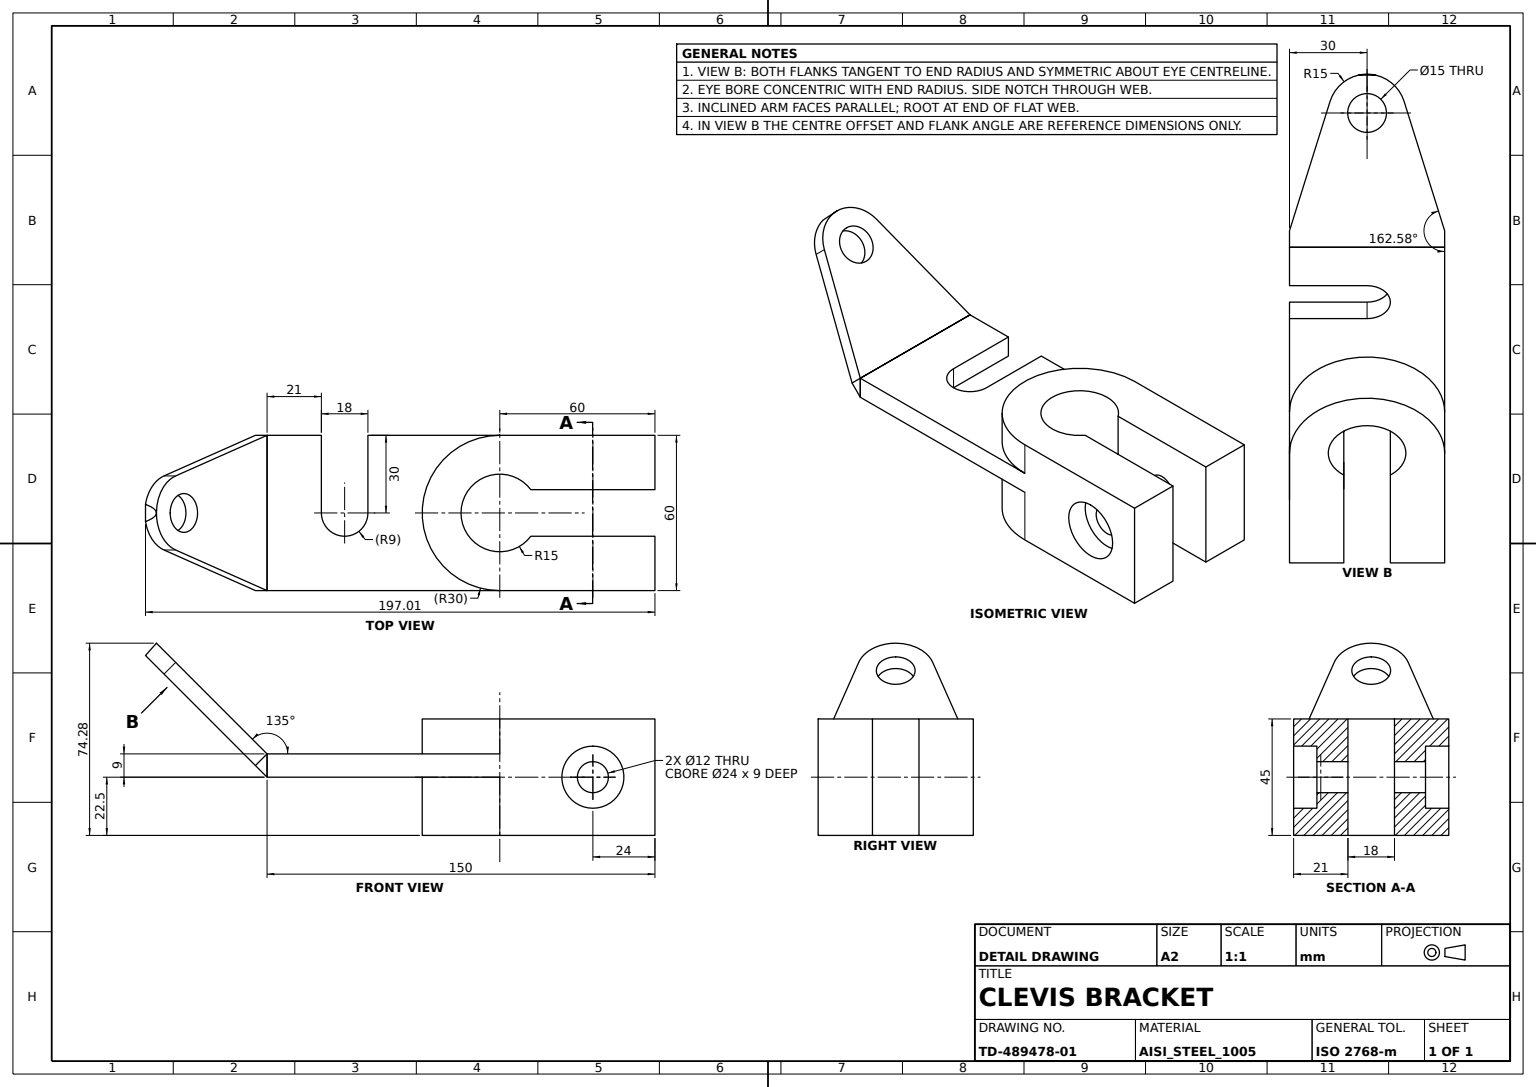
ISO-10303-21;
HEADER;
FILE_DESCRIPTION((''),'2;1');
FILE_NAME('','',(''),(''),'','','');
FILE_SCHEMA(('AUTOMOTIVE_DESIGN'));
ENDSEC;
DATA;
#1=APPLICATION_CONTEXT('');
#2=PRODUCT_CONTEXT('',#1,'mechanical');
#3=PRODUCT('','','',(#2));
#4=PRODUCT_DEFINITION_FORMATION('','',#3);
#5=PRODUCT_DEFINITION_CONTEXT('',#1,'design');
#6=PRODUCT_DEFINITION('','',#4,#5);
#7=PRODUCT_DEFINITION_SHAPE('','',#6);
#8=(LENGTH_UNIT()NAMED_UNIT(*)SI_UNIT(.MILLI.,.METRE.));
#9=(NAMED_UNIT(*)PLANE_ANGLE_UNIT()SI_UNIT($,.RADIAN.));
#10=(NAMED_UNIT(*)SI_UNIT($,.STERADIAN.)SOLID_ANGLE_UNIT());
#11=UNCERTAINTY_MEASURE_WITH_UNIT(LENGTH_MEASURE(0.005),#8,'distance_accuracy_value','');
#12=(GEOMETRIC_REPRESENTATION_CONTEXT(3)GLOBAL_UNCERTAINTY_ASSIGNED_CONTEXT((#11))GLOBAL_UNIT_ASSIGNED_CONTEXT((#8,#9,#10))REPRESENTATION_CONTEXT('',''));
#13=CARTESIAN_POINT('',(-90.,-30.,9.));
#14=VERTEX_POINT('',#13);
#15=CARTESIAN_POINT('',(-90.,30.,9.));
#16=VERTEX_POINT('',#15);
#17=DIRECTION('',(0.,1.,0.));
#18=VECTOR('',#17,1000.);
#19=LINE('',#13,#18);
#20=EDGE_CURVE('',#14,#16,#19,.T.);
#21=ORIENTED_EDGE('',*,*,#20,.F.);
#22=CARTESIAN_POINT('',(0.,-30.,9.));
#23=VERTEX_POINT('',#22);
#24=DIRECTION('',(-1.,0.,0.));
#25=VECTOR('',#24,1000.);
#26=LINE('',#22,#25);
#27=EDGE_CURVE('',#23,#14,#26,.T.);
#28=ORIENTED_EDGE('',*,*,#27,.F.);
#29=CARTESIAN_POINT('',(0.,30.,9.));
#30=VERTEX_POINT('',#29);
#31=CARTESIAN_POINT('',(0.,0.,9.));
#32=DIRECTION('',(0.,0.,1.));
#33=DIRECTION('',(1.,0.,0.));
#34=AXIS2_PLACEMENT_3D('',#31,#32,#33);
#35=CIRCLE('',#34,30.);
#36=EDGE_CURVE('',#30,#23,#35,.T.);
#37=ORIENTED_EDGE('',*,*,#36,.F.);
#38=CARTESIAN_POINT('',(-51.,30.,9.));
#39=VERTEX_POINT('',#38);
#40=VECTOR('',#33,1000.);
#41=LINE('',#38,#40);
#42=EDGE_CURVE('',#39,#30,#41,.T.);
#43=ORIENTED_EDGE('',*,*,#42,.F.);
#44=CARTESIAN_POINT('',(-51.,0.,9.));
#45=VERTEX_POINT('',#44);
#46=LINE('',#44,#18);
#47=EDGE_CURVE('',#45,#39,#46,.T.);
#48=ORIENTED_EDGE('',*,*,#47,.F.);
#49=CARTESIAN_POINT('',(-69.,0.,9.));
#50=VERTEX_POINT('',#49);
#51=CARTESIAN_POINT('',(-60.,0.,9.));
#52=AXIS2_PLACEMENT_3D('',#51,#32,#33);
#53=CIRCLE('',#52,9.);
#54=EDGE_CURVE('',#50,#45,#53,.T.);
#55=ORIENTED_EDGE('',*,*,#54,.F.);
#56=CARTESIAN_POINT('',(-69.,30.,9.));
#57=VERTEX_POINT('',#56);
#58=DIRECTION('',(0.,-1.,0.));
#59=VECTOR('',#58,1000.);
#60=LINE('',#56,#59);
#61=EDGE_CURVE('',#57,#50,#60,.T.);
#62=ORIENTED_EDGE('',*,*,#61,.F.);
#63=LINE('',#15,#40);
#64=EDGE_CURVE('',#16,#57,#63,.T.);
#65=ORIENTED_EDGE('',*,*,#64,.F.);
#66=EDGE_LOOP('',(#21,#28,#37,#43,#48,#55,#62,#65));
#67=FACE_BOUND('',#66,.T.);
#68=PLANE('',#52);
#69=ADVANCED_FACE('',(#67),#68,.T.);
#70=CARTESIAN_POINT('',(60.,-30.,22.5));
#71=VERTEX_POINT('',#70);
#72=CARTESIAN_POINT('',(60.,-30.,-22.5));
#73=VERTEX_POINT('',#72);
#74=DIRECTION('',(0.,0.,-1.));
#75=VECTOR('',#74,1000.);
#76=LINE('',#70,#75);
#77=EDGE_CURVE('',#71,#73,#76,.T.);
#78=ORIENTED_EDGE('',*,*,#77,.T.);
#79=CARTESIAN_POINT('',(60.,-9.,-22.5));
#80=VERTEX_POINT('',#79);
#81=LINE('',#72,#18);
#82=EDGE_CURVE('',#73,#80,#81,.T.);
#83=ORIENTED_EDGE('',*,*,#82,.T.);
#84=CARTESIAN_POINT('',(60.,-9.,22.5));
#85=VERTEX_POINT('',#84);
#86=LINE('',#84,#75);
#87=EDGE_CURVE('',#85,#80,#86,.T.);
#88=ORIENTED_EDGE('',*,*,#87,.F.);
#89=LINE('',#70,#18);
#90=EDGE_CURVE('',#71,#85,#89,.T.);
#91=ORIENTED_EDGE('',*,*,#90,.F.);
#92=EDGE_LOOP('',(#78,#83,#88,#91));
#93=FACE_BOUND('',#92,.T.);
#94=AXIS2_PLACEMENT_3D('',#70,#24,#58);
#95=PLANE('',#94);
#96=ADVANCED_FACE('',(#93),#95,.F.);
#97=CARTESIAN_POINT('',(36.,21.,-12.));
#98=VERTEX_POINT('',#97);
#99=CARTESIAN_POINT('',(36.,21.,0.));
#100=AXIS2_PLACEMENT_3D('',#99,#58,#74);
#101=CIRCLE('',#100,12.);
#102=EDGE_CURVE('',#98,#98,#101,.T.);
#103=ORIENTED_EDGE('',*,*,#102,.T.);
#104=EDGE_LOOP('',(#103));
#105=FACE_BOUND('',#104,.T.);
#106=CARTESIAN_POINT('',(36.,30.,-12.));
#107=VERTEX_POINT('',#106);
#108=CARTESIAN_POINT('',(36.,30.,0.));
#109=AXIS2_PLACEMENT_3D('',#108,#58,#74);
#110=CIRCLE('',#109,12.);
#111=EDGE_CURVE('',#107,#107,#110,.T.);
#112=ORIENTED_EDGE('',*,*,#111,.F.);
#113=EDGE_LOOP('',(#112));
#114=FACE_BOUND('',#113,.T.);
#115=CYLINDRICAL_SURFACE('',#109,12.);
#116=ADVANCED_FACE('',(#105,#114),#115,.F.);
#117=ORIENTED_EDGE('',*,*,#64,.T.);
#118=CARTESIAN_POINT('',(-69.,30.,0.));
#119=VERTEX_POINT('',#118);
#120=LINE('',#56,#75);
#121=EDGE_CURVE('',#57,#119,#120,.T.);
#122=ORIENTED_EDGE('',*,*,#121,.T.);
#123=CARTESIAN_POINT('',(-90.,30.,0.));
#124=VERTEX_POINT('',#123);
#125=LINE('',#123,#40);
#126=EDGE_CURVE('',#124,#119,#125,.T.);
#127=ORIENTED_EDGE('',*,*,#126,.F.);
#128=LINE('',#15,#75);
#129=EDGE_CURVE('',#16,#124,#128,.T.);
#130=ORIENTED_EDGE('',*,*,#129,.F.);
#131=EDGE_LOOP('',(#117,#122,#127,#130));
#132=FACE_BOUND('',#131,.T.);
#133=AXIS2_PLACEMENT_3D('',#15,#17,#24);
#134=PLANE('',#133);
#135=ADVANCED_FACE('',(#132),#134,.T.);
#136=CARTESIAN_POINT('',(36.,9.,6.));
#137=VERTEX_POINT('',#136);
#138=CARTESIAN_POINT('',(36.,9.,0.));
#139=AXIS2_PLACEMENT_3D('',#138,#17,#32);
#140=CIRCLE('',#139,6.);
#141=EDGE_CURVE('',#137,#137,#140,.T.);
#142=ORIENTED_EDGE('',*,*,#141,.F.);
#143=EDGE_LOOP('',(#142));
#144=FACE_BOUND('',#143,.T.);
#145=CARTESIAN_POINT('',(36.,21.,-6.));
#146=VERTEX_POINT('',#145);
#147=CIRCLE('',#100,6.);
#148=EDGE_CURVE('',#146,#146,#147,.T.);
#149=ORIENTED_EDGE('',*,*,#148,.F.);
#150=EDGE_LOOP('',(#149));
#151=FACE_BOUND('',#150,.T.);
#152=CARTESIAN_POINT('',(36.,-60.916439,0.));
#153=AXIS2_PLACEMENT_3D('',#152,#58,#74);
#154=CYLINDRICAL_SURFACE('',#153,6.);
#155=ADVANCED_FACE('',(#144,#151),#154,.F.);
#156=CARTESIAN_POINT('',(36.,-30.,12.));
#157=VERTEX_POINT('',#156);
#158=CARTESIAN_POINT('',(36.,-30.,0.));
#159=AXIS2_PLACEMENT_3D('',#158,#17,#32);
#160=CIRCLE('',#159,12.);
#161=EDGE_CURVE('',#157,#157,#160,.T.);
#162=ORIENTED_EDGE('',*,*,#161,.F.);
#163=EDGE_LOOP('',(#162));
#164=FACE_BOUND('',#163,.T.);
#165=CARTESIAN_POINT('',(36.,-21.,12.));
#166=VERTEX_POINT('',#165);
#167=CARTESIAN_POINT('',(36.,-21.,0.));
#168=AXIS2_PLACEMENT_3D('',#167,#17,#32);
#169=CIRCLE('',#168,12.);
#170=EDGE_CURVE('',#166,#166,#169,.F.);
#171=ORIENTED_EDGE('',*,*,#170,.F.);
#172=EDGE_LOOP('',(#171));
#173=FACE_BOUND('',#172,.T.);
#174=CYLINDRICAL_SURFACE('',#159,12.);
#175=ADVANCED_FACE('',(#164,#173),#174,.F.);
#176=CARTESIAN_POINT('',(0.,30.,-22.5));
#177=VERTEX_POINT('',#176);
#178=CARTESIAN_POINT('',(0.,-30.,-22.5));
#179=VERTEX_POINT('',#178);
#180=CARTESIAN_POINT('',(0.,0.,-22.5));
#181=AXIS2_PLACEMENT_3D('',#180,#32,#33);
#182=CIRCLE('',#181,30.);
#183=EDGE_CURVE('',#177,#179,#182,.T.);
#184=ORIENTED_EDGE('',*,*,#183,.T.);
#185=CARTESIAN_POINT('',(0.,-30.,0.));
#186=VERTEX_POINT('',#185);
#187=CARTESIAN_POINT('',(0.,-30.,22.5));
#188=LINE('',#187,#75);
#189=EDGE_CURVE('',#186,#179,#188,.T.);
#190=ORIENTED_EDGE('',*,*,#189,.F.);
#191=CARTESIAN_POINT('',(0.,30.,0.));
#192=VERTEX_POINT('',#191);
#193=CARTESIAN_POINT('',(0.,0.,0.));
#194=AXIS2_PLACEMENT_3D('',#193,#32,#33);
#195=CIRCLE('',#194,30.);
#196=EDGE_CURVE('',#192,#186,#195,.T.);
#197=ORIENTED_EDGE('',*,*,#196,.F.);
#198=CARTESIAN_POINT('',(0.,30.,22.5));
#199=LINE('',#198,#75);
#200=EDGE_CURVE('',#192,#177,#199,.T.);
#201=ORIENTED_EDGE('',*,*,#200,.T.);
#202=EDGE_LOOP('',(#184,#190,#197,#201));
#203=FACE_BOUND('',#202,.T.);
#204=CARTESIAN_POINT('',(0.,0.,22.5));
#205=AXIS2_PLACEMENT_3D('',#204,#74,#24);
#206=CYLINDRICAL_SURFACE('',#205,30.);
#207=ADVANCED_FACE('',(#203),#206,.T.);
#208=ORIENTED_EDGE('',*,*,#102,.F.);
#209=EDGE_LOOP('',(#208));
#210=FACE_BOUND('',#209,.T.);
#211=ORIENTED_EDGE('',*,*,#148,.T.);
#212=EDGE_LOOP('',(#211));
#213=FACE_BOUND('',#212,.T.);
#214=PLANE('',#100);
#215=ADVANCED_FACE('',(#210,#213),#214,.F.);
#216=ORIENTED_EDGE('',*,*,#170,.T.);
#217=EDGE_LOOP('',(#216));
#218=FACE_BOUND('',#217,.T.);
#219=CARTESIAN_POINT('',(36.,-21.,6.));
#220=VERTEX_POINT('',#219);
#221=CIRCLE('',#168,6.);
#222=EDGE_CURVE('',#220,#220,#221,.F.);
#223=ORIENTED_EDGE('',*,*,#222,.F.);
#224=EDGE_LOOP('',(#223));
#225=FACE_BOUND('',#224,.T.);
#226=PLANE('',#168);
#227=ADVANCED_FACE('',(#218,#225),#226,.F.);
#228=CARTESIAN_POINT('',(12.,9.,22.5));
#229=VERTEX_POINT('',#228);
#230=CARTESIAN_POINT('',(60.,9.,22.5));
#231=VERTEX_POINT('',#230);
#232=LINE('',#228,#40);
#233=EDGE_CURVE('',#229,#231,#232,.T.);
#234=ORIENTED_EDGE('',*,*,#233,.T.);
#235=CARTESIAN_POINT('',(60.,30.,22.5));
#236=VERTEX_POINT('',#235);
#237=LINE('',#230,#18);
#238=EDGE_CURVE('',#231,#236,#237,.T.);
#239=ORIENTED_EDGE('',*,*,#238,.T.);
#240=VERTEX_POINT('',#198);
#241=LINE('',#235,#25);
#242=EDGE_CURVE('',#236,#240,#241,.T.);
#243=ORIENTED_EDGE('',*,*,#242,.T.);
#244=VERTEX_POINT('',#187);
#245=AXIS2_PLACEMENT_3D('',#204,#32,#33);
#246=CIRCLE('',#245,30.);
#247=EDGE_CURVE('',#240,#244,#246,.T.);
#248=ORIENTED_EDGE('',*,*,#247,.T.);
#249=LINE('',#187,#40);
#250=EDGE_CURVE('',#244,#71,#249,.T.);
#251=ORIENTED_EDGE('',*,*,#250,.T.);
#252=ORIENTED_EDGE('',*,*,#90,.T.);
#253=CARTESIAN_POINT('',(12.,-9.,22.5));
#254=VERTEX_POINT('',#253);
#255=LINE('',#84,#25);
#256=EDGE_CURVE('',#85,#254,#255,.T.);
#257=ORIENTED_EDGE('',*,*,#256,.T.);
#258=AXIS2_PLACEMENT_3D('',#204,#74,#33);
#259=CIRCLE('',#258,15.);
#260=EDGE_CURVE('',#254,#229,#259,.T.);
#261=ORIENTED_EDGE('',*,*,#260,.T.);
#262=EDGE_LOOP('',(#234,#239,#243,#248,#251,#252,#257,#261));
#263=FACE_BOUND('',#262,.T.);
#264=PLANE('',#245);
#265=ADVANCED_FACE('',(#263),#264,.T.);
#266=ORIENTED_EDGE('',*,*,#20,.T.);
#267=ORIENTED_EDGE('',*,*,#129,.T.);
#268=CARTESIAN_POINT('',(-90.,-30.,0.));
#269=VERTEX_POINT('',#268);
#270=LINE('',#268,#18);
#271=EDGE_CURVE('',#269,#124,#270,.T.);
#272=ORIENTED_EDGE('',*,*,#271,.F.);
#273=LINE('',#13,#75);
#274=EDGE_CURVE('',#14,#269,#273,.T.);
#275=ORIENTED_EDGE('',*,*,#274,.F.);
#276=EDGE_LOOP('',(#266,#267,#272,#275));
#277=FACE_BOUND('',#276,.T.);
#278=AXIS2_PLACEMENT_3D('',#13,#24,#32);
#279=PLANE('',#278);
#280=ADVANCED_FACE('',(#277),#279,.T.);
#281=CARTESIAN_POINT('',(12.,9.,-22.5));
#282=VERTEX_POINT('',#281);
#283=LINE('',#228,#75);
#284=EDGE_CURVE('',#229,#282,#283,.T.);
#285=ORIENTED_EDGE('',*,*,#284,.T.);
#286=CARTESIAN_POINT('',(60.,9.,-22.5));
#287=VERTEX_POINT('',#286);
#288=LINE('',#281,#40);
#289=EDGE_CURVE('',#282,#287,#288,.T.);
#290=ORIENTED_EDGE('',*,*,#289,.T.);
#291=LINE('',#230,#75);
#292=EDGE_CURVE('',#231,#287,#291,.T.);
#293=ORIENTED_EDGE('',*,*,#292,.F.);
#294=ORIENTED_EDGE('',*,*,#233,.F.);
#295=EDGE_LOOP('',(#285,#290,#293,#294));
#296=FACE_BOUND('',#295,.T.);
#297=ORIENTED_EDGE('',*,*,#141,.T.);
#298=EDGE_LOOP('',(#297));
#299=FACE_BOUND('',#298,.T.);
#300=AXIS2_PLACEMENT_3D('',#228,#17,#32);
#301=PLANE('',#300);
#302=ADVANCED_FACE('',(#296,#299),#301,.F.);
#303=CARTESIAN_POINT('',(-51.,30.,0.));
#304=VERTEX_POINT('',#303);
#305=LINE('',#38,#75);
#306=EDGE_CURVE('',#39,#304,#305,.T.);
#307=ORIENTED_EDGE('',*,*,#306,.T.);
#308=CARTESIAN_POINT('',(-51.,0.,0.));
#309=VERTEX_POINT('',#308);
#310=LINE('',#308,#18);
#311=EDGE_CURVE('',#309,#304,#310,.T.);
#312=ORIENTED_EDGE('',*,*,#311,.F.);
#313=LINE('',#44,#75);
#314=EDGE_CURVE('',#45,#309,#313,.T.);
#315=ORIENTED_EDGE('',*,*,#314,.F.);
#316=ORIENTED_EDGE('',*,*,#47,.T.);
#317=EDGE_LOOP('',(#307,#312,#315,#316));
#318=FACE_BOUND('',#317,.T.);
#319=AXIS2_PLACEMENT_3D('',#44,#24,#58);
#320=PLANE('',#319);
#321=ADVANCED_FACE('',(#318),#320,.T.);
#322=ORIENTED_EDGE('',*,*,#306,.F.);
#323=ORIENTED_EDGE('',*,*,#42,.T.);
#324=EDGE_CURVE('',#240,#30,#199,.T.);
#325=ORIENTED_EDGE('',*,*,#324,.F.);
#326=ORIENTED_EDGE('',*,*,#242,.F.);
#327=CARTESIAN_POINT('',(60.,30.,-22.5));
#328=VERTEX_POINT('',#327);
#329=LINE('',#235,#75);
#330=EDGE_CURVE('',#236,#328,#329,.T.);
#331=ORIENTED_EDGE('',*,*,#330,.T.);
#332=LINE('',#327,#25);
#333=EDGE_CURVE('',#328,#177,#332,.T.);
#334=ORIENTED_EDGE('',*,*,#333,.T.);
#335=ORIENTED_EDGE('',*,*,#200,.F.);
#336=LINE('',#303,#40);
#337=EDGE_CURVE('',#304,#192,#336,.T.);
#338=ORIENTED_EDGE('',*,*,#337,.F.);
#339=EDGE_LOOP('',(#322,#323,#325,#326,#331,#334,#335,#338));
#340=FACE_BOUND('',#339,.T.);
#341=ORIENTED_EDGE('',*,*,#111,.T.);
#342=EDGE_LOOP('',(#341));
#343=FACE_BOUND('',#342,.T.);
#344=AXIS2_PLACEMENT_3D('',#235,#58,#74);
#345=PLANE('',#344);
#346=ADVANCED_FACE('',(#340,#343),#345,.F.);
#347=ORIENTED_EDGE('',*,*,#54,.T.);
#348=ORIENTED_EDGE('',*,*,#314,.T.);
#349=CARTESIAN_POINT('',(-69.,0.,0.));
#350=VERTEX_POINT('',#349);
#351=CARTESIAN_POINT('',(-60.,0.,0.));
#352=AXIS2_PLACEMENT_3D('',#351,#32,#33);
#353=CIRCLE('',#352,9.);
#354=EDGE_CURVE('',#350,#309,#353,.T.);
#355=ORIENTED_EDGE('',*,*,#354,.F.);
#356=LINE('',#49,#75);
#357=EDGE_CURVE('',#50,#350,#356,.T.);
#358=ORIENTED_EDGE('',*,*,#357,.F.);
#359=EDGE_LOOP('',(#347,#348,#355,#358));
#360=FACE_BOUND('',#359,.T.);
#361=AXIS2_PLACEMENT_3D('',#51,#74,#24);
#362=CYLINDRICAL_SURFACE('',#361,9.);
#363=ADVANCED_FACE('',(#360),#362,.F.);
#364=ORIENTED_EDGE('',*,*,#284,.F.);
#365=ORIENTED_EDGE('',*,*,#260,.F.);
#366=CARTESIAN_POINT('',(12.,-9.,-22.5));
#367=VERTEX_POINT('',#366);
#368=LINE('',#253,#75);
#369=EDGE_CURVE('',#254,#367,#368,.T.);
#370=ORIENTED_EDGE('',*,*,#369,.T.);
#371=AXIS2_PLACEMENT_3D('',#180,#74,#33);
#372=CIRCLE('',#371,15.);
#373=EDGE_CURVE('',#367,#282,#372,.T.);
#374=ORIENTED_EDGE('',*,*,#373,.T.);
#375=EDGE_LOOP('',(#364,#365,#370,#374));
#376=FACE_BOUND('',#375,.T.);
#377=CYLINDRICAL_SURFACE('',#205,15.);
#378=ADVANCED_FACE('',(#376),#377,.F.);
#379=ORIENTED_EDGE('',*,*,#121,.F.);
#380=ORIENTED_EDGE('',*,*,#61,.T.);
#381=ORIENTED_EDGE('',*,*,#357,.T.);
#382=LINE('',#118,#59);
#383=EDGE_CURVE('',#119,#350,#382,.T.);
#384=ORIENTED_EDGE('',*,*,#383,.F.);
#385=EDGE_LOOP('',(#379,#380,#381,#384));
#386=FACE_BOUND('',#385,.T.);
#387=AXIS2_PLACEMENT_3D('',#56,#33,#74);
#388=PLANE('',#387);
#389=ADVANCED_FACE('',(#386),#388,.T.);
#390=ORIENTED_EDGE('',*,*,#337,.T.);
#391=ORIENTED_EDGE('',*,*,#196,.T.);
#392=LINE('',#185,#25);
#393=EDGE_CURVE('',#186,#269,#392,.T.);
#394=ORIENTED_EDGE('',*,*,#393,.T.);
#395=ORIENTED_EDGE('',*,*,#271,.T.);
#396=ORIENTED_EDGE('',*,*,#126,.T.);
#397=ORIENTED_EDGE('',*,*,#383,.T.);
#398=ORIENTED_EDGE('',*,*,#354,.T.);
#399=ORIENTED_EDGE('',*,*,#311,.T.);
#400=EDGE_LOOP('',(#390,#391,#394,#395,#396,#397,#398,#399));
#401=FACE_BOUND('',#400,.T.);
#402=PLANE('',#352);
#403=ADVANCED_FACE('',(#401),#402,.F.);
#404=ORIENTED_EDGE('',*,*,#289,.F.);
#405=ORIENTED_EDGE('',*,*,#373,.F.);
#406=LINE('',#79,#25);
#407=EDGE_CURVE('',#80,#367,#406,.T.);
#408=ORIENTED_EDGE('',*,*,#407,.F.);
#409=ORIENTED_EDGE('',*,*,#82,.F.);
#410=LINE('',#178,#40);
#411=EDGE_CURVE('',#179,#73,#410,.T.);
#412=ORIENTED_EDGE('',*,*,#411,.F.);
#413=ORIENTED_EDGE('',*,*,#183,.F.);
#414=ORIENTED_EDGE('',*,*,#333,.F.);
#415=LINE('',#286,#18);
#416=EDGE_CURVE('',#287,#328,#415,.T.);
#417=ORIENTED_EDGE('',*,*,#416,.F.);
#418=EDGE_LOOP('',(#404,#405,#408,#409,#412,#413,#414,#417));
#419=FACE_BOUND('',#418,.T.);
#420=PLANE('',#181);
#421=ADVANCED_FACE('',(#419),#420,.F.);
#422=ORIENTED_EDGE('',*,*,#247,.F.);
#423=ORIENTED_EDGE('',*,*,#324,.T.);
#424=ORIENTED_EDGE('',*,*,#36,.T.);
#425=EDGE_CURVE('',#244,#23,#188,.T.);
#426=ORIENTED_EDGE('',*,*,#425,.F.);
#427=EDGE_LOOP('',(#422,#423,#424,#426));
#428=FACE_BOUND('',#427,.T.);
#429=ADVANCED_FACE('',(#428),#206,.T.);
#430=ORIENTED_EDGE('',*,*,#407,.T.);
#431=ORIENTED_EDGE('',*,*,#369,.F.);
#432=ORIENTED_EDGE('',*,*,#256,.F.);
#433=ORIENTED_EDGE('',*,*,#87,.T.);
#434=EDGE_LOOP('',(#430,#431,#432,#433));
#435=FACE_BOUND('',#434,.T.);
#436=CARTESIAN_POINT('',(36.,-9.,-6.));
#437=VERTEX_POINT('',#436);
#438=CARTESIAN_POINT('',(36.,-9.,0.));
#439=AXIS2_PLACEMENT_3D('',#438,#58,#74);
#440=CIRCLE('',#439,6.);
#441=EDGE_CURVE('',#437,#437,#440,.T.);
#442=ORIENTED_EDGE('',*,*,#441,.T.);
#443=EDGE_LOOP('',(#442));
#444=FACE_BOUND('',#443,.T.);
#445=AXIS2_PLACEMENT_3D('',#84,#58,#74);
#446=PLANE('',#445);
#447=ADVANCED_FACE('',(#435,#444),#446,.F.);
#448=ORIENTED_EDGE('',*,*,#425,.T.);
#449=ORIENTED_EDGE('',*,*,#27,.T.);
#450=ORIENTED_EDGE('',*,*,#274,.T.);
#451=ORIENTED_EDGE('',*,*,#393,.F.);
#452=ORIENTED_EDGE('',*,*,#189,.T.);
#453=ORIENTED_EDGE('',*,*,#411,.T.);
#454=ORIENTED_EDGE('',*,*,#77,.F.);
#455=ORIENTED_EDGE('',*,*,#250,.F.);
#456=EDGE_LOOP('',(#448,#449,#450,#451,#452,#453,#454,#455));
#457=FACE_BOUND('',#456,.T.);
#458=ORIENTED_EDGE('',*,*,#161,.T.);
#459=EDGE_LOOP('',(#458));
#460=FACE_BOUND('',#459,.T.);
#461=AXIS2_PLACEMENT_3D('',#187,#17,#32);
#462=PLANE('',#461);
#463=ADVANCED_FACE('',(#457,#460),#462,.F.);
#464=ORIENTED_EDGE('',*,*,#222,.T.);
#465=EDGE_LOOP('',(#464));
#466=FACE_BOUND('',#465,.T.);
#467=ORIENTED_EDGE('',*,*,#441,.F.);
#468=EDGE_LOOP('',(#467));
#469=FACE_BOUND('',#468,.T.);
#470=CARTESIAN_POINT('',(36.,60.916439,0.));
#471=AXIS2_PLACEMENT_3D('',#470,#17,#32);
#472=CYLINDRICAL_SURFACE('',#471,6.);
#473=ADVANCED_FACE('',(#466,#469),#472,.F.);
#474=ORIENTED_EDGE('',*,*,#330,.F.);
#475=ORIENTED_EDGE('',*,*,#238,.F.);
#476=ORIENTED_EDGE('',*,*,#292,.T.);
#477=ORIENTED_EDGE('',*,*,#416,.T.);
#478=EDGE_LOOP('',(#474,#475,#476,#477));
#479=FACE_BOUND('',#478,.T.);
#480=AXIS2_PLACEMENT_3D('',#230,#24,#58);
#481=PLANE('',#480);
#482=ADVANCED_FACE('',(#479),#481,.F.);
#483=CLOSED_SHELL('',(#69,#96,#116,#135,#155,#175,#207,#215,#227,#265,#280,#302,#321,#346,#363,#378,#389,#403,#421,#429,#447,#463,#473,#482));
#484=MANIFOLD_SOLID_BREP('',#483);
#485=CARTESIAN_POINT('',(-125.349193,14.311818,44.349193));
#486=VERTEX_POINT('',#485);
#487=CARTESIAN_POINT('',(-129.849193,14.311818,39.849193));
#488=VERTEX_POINT('',#487);
#489=CARTESIAN_POINT('',(-167.7756,14.311818,1.922787));
#490=DIRECTION('',(0.707106781,0.,0.707106781));
#491=VECTOR('',#490,1000.);
#492=LINE('',#489,#491);
#493=EDGE_CURVE('',#486,#488,#492,.F.);
#494=ORIENTED_EDGE('',*,*,#493,.F.);
#495=VERTEX_POINT('',#15);
#496=DIRECTION('',(0.674665588,0.299420588,-0.674665588));
#497=VECTOR('',#496,1000.);
#498=LINE('',#485,#497);
#499=EDGE_CURVE('',#486,#495,#498,.T.);
#500=ORIENTED_EDGE('',*,*,#499,.T.);
#501=CARTESIAN_POINT('',(-94.5,30.,4.5));
#502=VERTEX_POINT('',#501);
#503=CARTESIAN_POINT('',(-132.426407,30.,-33.426407));
#504=LINE('',#503,#491);
#505=EDGE_CURVE('',#502,#495,#504,.T.);
#506=ORIENTED_EDGE('',*,*,#505,.F.);
#507=CARTESIAN_POINT('',(-90.403437,31.818079,0.403437));
#508=LINE('',#507,#497);
#509=EDGE_CURVE('',#488,#502,#508,.T.);
#510=ORIENTED_EDGE('',*,*,#509,.F.);
#511=EDGE_LOOP('',(#494,#500,#506,#510));
#512=FACE_BOUND('',#511,.T.);
#513=DIRECTION('',(0.211722328,-0.954121225,-0.211722328));
#514=DIRECTION('',(0.976253017,0.216633438,0.));
#515=AXIS2_PLACEMENT_3D('',#489,#513,#514);
#516=PLANE('',#515);
#517=ADVANCED_FACE('',(#512),#516,.F.);
#518=CARTESIAN_POINT('',(-127.476659,0.,46.476659));
#519=VERTEX_POINT('',#518);
#520=CARTESIAN_POINT('',(-122.173359,0.,41.173359));
#521=DIRECTION('',(-0.707106781,0.,0.707106781));
#522=AXIS2_PLACEMENT_3D('',#520,#490,#521);
#523=CIRCLE('',#522,7.5);
#524=EDGE_CURVE('',#519,#519,#523,.T.);
#525=ORIENTED_EDGE('',*,*,#524,.F.);
#526=EDGE_LOOP('',(#525));
#527=FACE_BOUND('',#526,.T.);
#528=VERTEX_POINT('',#13);
#529=LINE('',#15,#59);
#530=EDGE_CURVE('',#495,#528,#529,.T.);
#531=ORIENTED_EDGE('',*,*,#530,.F.);
#532=ORIENTED_EDGE('',*,*,#499,.F.);
#533=CARTESIAN_POINT('',(-132.77996,0.,51.77996));
#534=VERTEX_POINT('',#533);
#535=DIRECTION('',(-0.707106781,0.,-0.707106781));
#536=AXIS2_PLACEMENT_3D('',#520,#535,#17);
#537=CIRCLE('',#536,15.);
#538=EDGE_CURVE('',#534,#486,#537,.T.);
#539=ORIENTED_EDGE('',*,*,#538,.F.);
#540=CARTESIAN_POINT('',(-125.349193,-14.311818,44.349193));
#541=VERTEX_POINT('',#540);
#542=EDGE_CURVE('',#541,#534,#537,.T.);
#543=ORIENTED_EDGE('',*,*,#542,.F.);
#544=DIRECTION('',(-0.674665588,0.299420588,0.674665588));
#545=VECTOR('',#544,1000.);
#546=LINE('',#13,#545);
#547=EDGE_CURVE('',#528,#541,#546,.T.);
#548=ORIENTED_EDGE('',*,*,#547,.F.);
#549=EDGE_LOOP('',(#531,#532,#539,#543,#548));
#550=FACE_BOUND('',#549,.T.);
#551=CARTESIAN_POINT('',(-132.77996,30.,51.77996));
#552=AXIS2_PLACEMENT_3D('',#551,#535,#521);
#553=PLANE('',#552);
#554=ADVANCED_FACE('',(#527,#550),#553,.F.);
#555=CARTESIAN_POINT('',(-129.849193,-14.311818,39.849193));
#556=VERTEX_POINT('',#555);
#557=CARTESIAN_POINT('',(-137.013302,-3.342323,47.013302));
#558=VERTEX_POINT('',#557);
#559=CARTESIAN_POINT('',(-126.673359,0.,36.673359));
#560=DIRECTION('',(0.707106781,0.,-0.707106781));
#561=AXIS2_PLACEMENT_3D('',#559,#490,#560);
#562=CIRCLE('',#561,15.);
#563=EDGE_CURVE('',#556,#558,#562,.F.);
#564=ORIENTED_EDGE('',*,*,#563,.T.);
#565=CARTESIAN_POINT('',(-137.013302,3.342323,47.013302));
#566=VERTEX_POINT('',#565);
#567=CARTESIAN_POINT('',(-137.013302,30.,47.013302));
#568=LINE('',#567,#59);
#569=EDGE_CURVE('',#566,#558,#568,.T.);
#570=ORIENTED_EDGE('',*,*,#569,.F.);
#571=EDGE_CURVE('',#566,#488,#562,.F.);
#572=ORIENTED_EDGE('',*,*,#571,.T.);
#573=ORIENTED_EDGE('',*,*,#509,.T.);
#574=VERTEX_POINT('',#123);
#575=VECTOR('',#521,1000.);
#576=LINE('',#123,#575);
#577=EDGE_CURVE('',#574,#502,#576,.T.);
#578=ORIENTED_EDGE('',*,*,#577,.F.);
#579=VERTEX_POINT('',#268);
#580=LINE('',#123,#59);
#581=EDGE_CURVE('',#574,#579,#580,.T.);
#582=ORIENTED_EDGE('',*,*,#581,.T.);
#583=CARTESIAN_POINT('',(-94.5,-30.,4.5));
#584=VERTEX_POINT('',#583);
#585=LINE('',#268,#575);
#586=EDGE_CURVE('',#579,#584,#585,.T.);
#587=ORIENTED_EDGE('',*,*,#586,.T.);
#588=CARTESIAN_POINT('',(-102.523963,-26.438918,12.523963));
#589=LINE('',#588,#545);
#590=EDGE_CURVE('',#584,#556,#589,.T.);
#591=ORIENTED_EDGE('',*,*,#590,.T.);
#592=EDGE_LOOP('',(#564,#570,#572,#573,#578,#582,#587,#591));
#593=FACE_BOUND('',#592,.T.);
#594=CARTESIAN_POINT('',(-121.370058,0.,31.370058));
#595=VERTEX_POINT('',#594);
#596=CIRCLE('',#561,7.5);
#597=EDGE_CURVE('',#595,#595,#596,.T.);
#598=ORIENTED_EDGE('',*,*,#597,.T.);
#599=EDGE_LOOP('',(#598));
#600=FACE_BOUND('',#599,.T.);
#601=AXIS2_PLACEMENT_3D('',#123,#490,#560);
#602=PLANE('',#601);
#603=ADVANCED_FACE('',(#593,#600),#602,.F.);
#604=EDGE_CURVE('',#495,#574,#128,.T.);
#605=ORIENTED_EDGE('',*,*,#604,.T.);
#606=ORIENTED_EDGE('',*,*,#577,.T.);
#607=ORIENTED_EDGE('',*,*,#505,.T.);
#608=EDGE_LOOP('',(#605,#606,#607));
#609=FACE_BOUND('',#608,.T.);
#610=AXIS2_PLACEMENT_3D('',#191,#58,#74);
#611=PLANE('',#610);
#612=ADVANCED_FACE('',(#609),#611,.F.);
#613=ORIENTED_EDGE('',*,*,#597,.F.);
#614=EDGE_LOOP('',(#613));
#615=FACE_BOUND('',#614,.T.);
#616=ORIENTED_EDGE('',*,*,#524,.T.);
#617=EDGE_LOOP('',(#616));
#618=FACE_BOUND('',#617,.T.);
#619=CARTESIAN_POINT('',(-164.599765,0.,-1.253048));
#620=AXIS2_PLACEMENT_3D('',#619,#490,#560);
#621=CYLINDRICAL_SURFACE('',#620,7.5);
#622=ADVANCED_FACE('',(#615,#618),#621,.F.);
#623=ORIENTED_EDGE('',*,*,#563,.F.);
#624=CARTESIAN_POINT('',(-167.7756,-14.311818,1.922787));
#625=LINE('',#624,#491);
#626=EDGE_CURVE('',#541,#556,#625,.F.);
#627=ORIENTED_EDGE('',*,*,#626,.F.);
#628=ORIENTED_EDGE('',*,*,#542,.T.);
#629=CARTESIAN_POINT('',(-301.165709,0.,-137.818992));
#630=DIRECTION('',(0.747696423,0.,-0.664040706));
#631=DIRECTION('',(0.664040706,0.,0.747696423));
#632=AXIS2_PLACEMENT_3D('',#629,#630,#631);
#633=ELLIPSE('',#632,253.577449,15.);
#634=EDGE_CURVE('',#558,#534,#633,.F.);
#635=ORIENTED_EDGE('',*,*,#634,.F.);
#636=EDGE_LOOP('',(#623,#627,#628,#635));
#637=FACE_BOUND('',#636,.T.);
#638=CYLINDRICAL_SURFACE('',#620,15.);
#639=ADVANCED_FACE('',(#637),#638,.T.);
#640=ORIENTED_EDGE('',*,*,#530,.T.);
#641=EDGE_CURVE('',#528,#579,#273,.T.);
#642=ORIENTED_EDGE('',*,*,#641,.T.);
#643=ORIENTED_EDGE('',*,*,#581,.F.);
#644=ORIENTED_EDGE('',*,*,#604,.F.);
#645=EDGE_LOOP('',(#640,#642,#643,#644));
#646=FACE_BOUND('',#645,.T.);
#647=AXIS2_PLACEMENT_3D('',#15,#24,#32);
#648=PLANE('',#647);
#649=ADVANCED_FACE('',(#646),#648,.F.);
#650=ORIENTED_EDGE('',*,*,#634,.T.);
#651=EDGE_CURVE('',#534,#566,#633,.F.);
#652=ORIENTED_EDGE('',*,*,#651,.T.);
#653=ORIENTED_EDGE('',*,*,#569,.T.);
#654=EDGE_LOOP('',(#650,#652,#653));
#655=FACE_BOUND('',#654,.T.);
#656=DIRECTION('',(-0.664040706,0.,-0.747696423));
#657=AXIS2_PLACEMENT_3D('',#567,#630,#656);
#658=PLANE('',#657);
#659=ADVANCED_FACE('',(#655),#658,.F.);
#660=CARTESIAN_POINT('',(-132.426407,-30.,-33.426407));
#661=LINE('',#660,#491);
#662=EDGE_CURVE('',#584,#528,#661,.T.);
#663=ORIENTED_EDGE('',*,*,#662,.T.);
#664=ORIENTED_EDGE('',*,*,#547,.T.);
#665=ORIENTED_EDGE('',*,*,#626,.T.);
#666=ORIENTED_EDGE('',*,*,#590,.F.);
#667=EDGE_LOOP('',(#663,#664,#665,#666));
#668=FACE_BOUND('',#667,.T.);
#669=DIRECTION('',(0.211722328,0.954121225,-0.211722328));
#670=DIRECTION('',(-0.976253017,0.216633438,0.));
#671=AXIS2_PLACEMENT_3D('',#660,#669,#670);
#672=PLANE('',#671);
#673=ADVANCED_FACE('',(#668),#672,.F.);
#674=ORIENTED_EDGE('',*,*,#641,.F.);
#675=ORIENTED_EDGE('',*,*,#662,.F.);
#676=ORIENTED_EDGE('',*,*,#586,.F.);
#677=EDGE_LOOP('',(#674,#675,#676));
#678=FACE_BOUND('',#677,.T.);
#679=AXIS2_PLACEMENT_3D('',#185,#58,#74);
#680=PLANE('',#679);
#681=ADVANCED_FACE('',(#678),#680,.T.);
#682=ORIENTED_EDGE('',*,*,#571,.F.);
#683=ORIENTED_EDGE('',*,*,#651,.F.);
#684=ORIENTED_EDGE('',*,*,#538,.T.);
#685=ORIENTED_EDGE('',*,*,#493,.T.);
#686=EDGE_LOOP('',(#682,#683,#684,#685));
#687=FACE_BOUND('',#686,.T.);
#688=ADVANCED_FACE('',(#687),#638,.T.);
#689=CLOSED_SHELL('',(#517,#554,#603,#612,#622,#639,#649,#659,#673,#681,#688));
#690=MANIFOLD_SOLID_BREP('',#689);
#691=ADVANCED_BREP_SHAPE_REPRESENTATION('',(#484,#690),#12);
#692=SHAPE_DEFINITION_REPRESENTATION(#7,#691);
ENDSEC;
END-ISO-10303-21;
